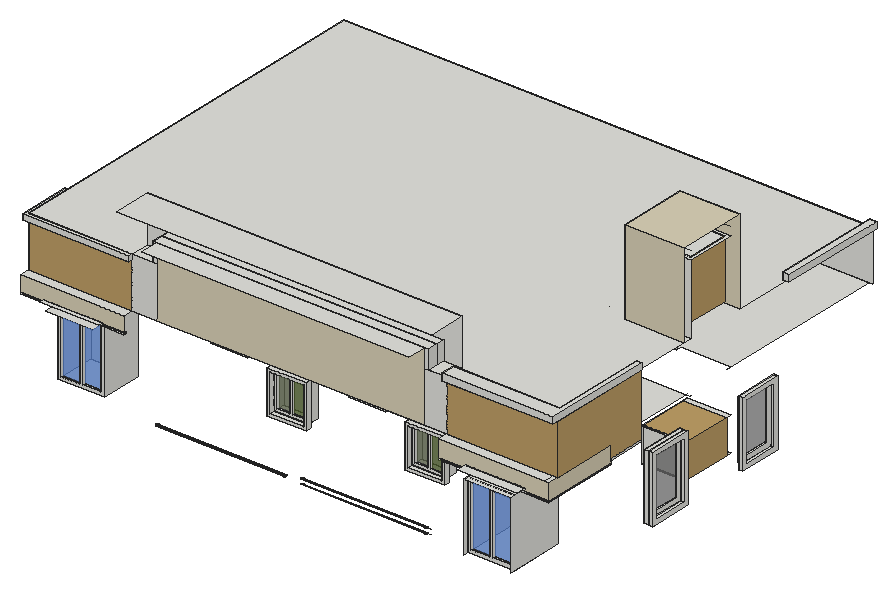
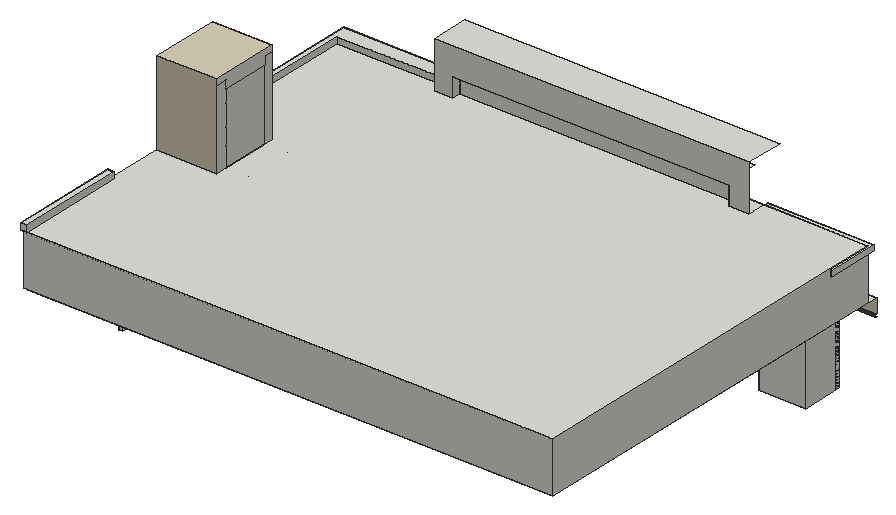
# SketchUp Ruby script. Lengths in inches.
U = 1.inch
M = Sketchup.active_model
def pt(a) = Geom::Point3d.new(a.map { |v| v * U })
def face(e, loops, mat)
  f = e.add_face(loops[0].map { |a| pt(a) })
  loops[1..].each { |l| e.add_face(l.map { |a| pt(a) }).erase! }
  f.material = f.back_material = mat if mat
  f
end
# faces: each face lists its corners as indices into pts; further lists are holes
def faces(e, pts, list, mat = nil) = list.each { |f| face(e, (f[0].is_a?(Array) ? f : [f]).map { |l| l.map { |i| pts[i] } }, mat) }
# xy, xz, yz: faces in a plane at the given z, y or x. An outline is a flat list of corners, or four numbers for a rectangle; further outlines are holes
def ring(l) = l.size == 4 ? [[l[0], l[1]], [l[2], l[1]], [l[2], l[3]], [l[0], l[3]]] : l.each_slice(2).to_a
def flat(e, list, mat, &to3) = list.each { |f| face(e, (f[0].is_a?(Array) ? f : [f]).map { |l| ring(l).map { |u, v| to3.(u, v) } }, mat) }
def xy(e, z, list, mat = nil) = flat(e, list, mat) { |x, y| [x, y, z] }
def xz(e, y, list, mat = nil) = flat(e, list, mat) { |x, z| [x, y, z] }
def yz(e, x, list, mat = nil) = flat(e, list, mat) { |y, z| [x, y, z] }
def lines(e, pts, list) = list.each { |a, b| e.add_line(pt(pts[a]), pt(pts[b])) }
# prism: a flat outline (further loops are holes) pulled along v
def prism(e, loops, v, mat = nil)
  f = face(e, loops, mat); d = Geom::Vector3d.new(v.map { |x| x * U })
  f.pushpull(f.normal.samedirection?(d) ? d.length : -d.length)
end
def box(e, o, s, mat = nil) = prism(e, [[o, [o[0] + s[0], o[1], o[2]], [o[0] + s[0], o[1] + s[1], o[2]], [o[0], o[1] + s[1], o[2]]]], [0, 0, s[2]], mat)
def at(x, y, z, deg = 0) = Geom::Transformation.translation(pt([x, y, z])) * Geom::Transformation.rotation(ORIGIN, Z_AXIS, deg.degrees)
def axes(o, x, y, z) = Geom::Transformation.new([*x, 0, *y, 0, *z, 0, *pt(o).to_a, 1])
def part(name) = M.definitions.add(name)
# library, detail: a bought-in or finely detailed component or shape, given as its bounding box
def library(name, o, s) = part(name).tap { |d| box(d.entities, o, s) }
def detail(e, o, s) = box(e.add_group.entities, o, s)
def put(e, d, t, mat = nil) = e.add_instance(d, t).tap { |i| i.material = mat if mat }
def group(e, t, mat = nil) = e.add_group.tap { |g| g.transformation = t; g.material = mat if mat }.entities
root = M.entities
M.materials.add("Generic").color = [191, 159, 103]
M.materials.add("Generic\#3").color = [218, 209, 183]
M.materials.add("[Color M06]").color = [86, 86, 86]
M.materials.add("[Translucent Glass Blue]").color = [100, 149, 237]
M.materials["[Translucent Glass Blue]"].alpha = 0.5
M.materials.add("[Translucent Glass Dark Green]").color = [62, 91, 5]
M.materials["[Translucent Glass Dark Green]"].alpha = 0.5
M.materials.add("[Translucent Glass Gray]").color = [128, 128, 128]
M.materials["[Translucent Glass Gray]"].alpha = 0.5
c1 = part("Group\#7")
xy(c1.entities,0,[[0,0,6,54.3125]])
xy(c1.entities,5.9,[[3,5.9,6,48.41]])
xy(c1.entities,81.98,[[3,5.9,6,48.41]])
xy(c1.entities,87.88,[[0,0,6,54.3125]])
xz(c1.entities,0,[[0,0,6,87.88]])
xz(c1.entities,5.9,[[3,5.9,6,81.98]])
xz(c1.entities,48.41,[[3,5.9,6,81.98]])
xz(c1.entities,54.3125,[[0,0,6,87.88]])
yz(c1.entities,0,[[0,0,54.3125,87.88]],"[Translucent Glass Gray]")
yz(c1.entities,3,[[5.9,5.9,48.41,81.98]],"[Translucent Glass Gray]")
yz(c1.entities,6,[[[0,0,54.3125,87.88],[5.9,5.9,48.41,81.98]]])
c2 = part("Group\#1")
xy(c2.entities,0,[[0,0,71.4375,6]])
xy(c2.entities,5.26,[[5.26,0,33.09,3],[38.35,0,66.18,3]])
xy(c2.entities,97.49,[[5.26,0,33.09,3],[38.35,0,66.18,3]])
xy(c2.entities,102.75,[[0,0,71.4375,6]])
xz(c2.entities,0,[[[0,0,71.4375,102.75],[38.35,5.26,66.18,97.49],[5.26,5.26,33.09,97.49]]])
xz(c2.entities,3,[[5.26,5.26,33.09,97.49],[38.35,5.26,66.18,97.49]],"[Translucent Glass Blue]")
xz(c2.entities,6,[[0,0,71.4375,102.75]],"[Translucent Glass Blue]")
yz(c2.entities,0,[[0,0,6,102.75]])
yz(c2.entities,5.26,[[0,5.26,3,97.49]])
yz(c2.entities,33.09,[[0,5.26,3,97.49]])
yz(c2.entities,38.35,[[0,5.26,3,97.49]])
yz(c2.entities,66.18,[[0,5.26,3,97.49]])
yz(c2.entities,71.4375,[[0,0,6,102.75]])
c3 = part("Group\#3")
xy(c3.entities,0,[[0,0,51.8125,6]])
xy(c3.entities,4.04,[[4.04,0,23.89,3],[27.93,0,47.77,3]])
xy(c3.entities,53.71,[[4.04,0,23.89,3],[27.93,0,47.77,3]])
xy(c3.entities,57.75,[[0,0,51.8125,6]])
xz(c3.entities,0,[[[0,0,51.8125,57.75],[4.04,4.04,23.89,53.71],[27.93,4.04,47.77,53.71]]])
xz(c3.entities,3,[[4.04,4.04,23.89,53.71],[27.93,4.04,47.77,53.71]],"[Translucent Glass Dark Green]")
xz(c3.entities,6,[[0,0,51.8125,57.75]],"[Translucent Glass Gray]")
yz(c3.entities,0,[[0,0,6,57.75]])
yz(c3.entities,4.04,[[0,4.04,3,53.71]])
yz(c3.entities,23.89,[[0,4.04,3,53.71]])
yz(c3.entities,27.93,[[0,4.04,3,53.71]])
yz(c3.entities,47.77,[[0,4.04,3,53.71]])
yz(c3.entities,51.8125,[[0,0,6,57.75]])
xy(root,918.09,[[802.875,257.24,809.375,324.36],[809.375,257.24,815.3125,324.36],[809.375,428.47,815.3125,495.59]])
xy(root,924.5,[[802.875,263.64,809.375,317.96],[809.375,263.64,815.3125,317.96],[802.875,434.88,809.375,489.19],[809.375,434.88,815.3125,489.19]])
xy(root,926.06,[[691.41,60.5625,762.85,142.1875]])
xy(root,926.27,[[49.01,83.8125,120.45,146.5625]])
xy(root,940.24,[[314.35,150.125,374.25,158.75],[524.6,150.125,584.5,158.75]])
xy(root,941.3,[[736.34,335.75,802.875,338.625],[736.34,413.6875,802.875,422.3125]])
xy(root,941.3,[[736.34,338.625,802.875,413.6875]],"Generic")
xy(root,944.28,[[318.39,150.125,370.21,158.75],[528.64,150.125,580.46,158.75],[318.39,158.75,370.21,177.1875],[528.64,158.75,580.46,177.1875]])
xy(root,993.42,[[736.34,335.75,802.875,338.625],[736.34,413.6875,802.875,422.3125]])
xy(root,993.42,[[736.34,338.625,802.875,413.6875]],"Generic")
xy(root,1002.03,[[318.39,150.125,370.21,158.75],[528.64,150.125,580.46,158.75],[318.39,158.75,370.21,177.1875],[528.64,158.75,580.46,177.1875]])
xy(root,1003,[[222.01,158.75,277.69,214.75],[432.26,158.75,487.94,214.75]])
xy(root,1006.07,[[314.35,150.125,374.25,158.75],[524.6,150.125,584.5,158.75]])
xy(root,1012.38,[[802.875,263.64,809.375,317.96],[809.375,263.64,815.3125,317.96],[802.875,434.88,809.375,489.19],[809.375,434.88,815.3125,489.19]])
xy(root,1018.78,[[802.875,257.24,809.375,324.36],[809.375,257.24,815.3125,324.36],[809.375,428.47,815.3125,495.59]])
xy(root,1028.81,[[691.41,53.22,762.85,142.1875]])
xy(root,1029.07,[[49.01,60.5625,120.45,83.8125],[49.01,83.8125,120.45,146.5625]])
xy(root,1031.12,[[641.55,68.5,682.51,69.9375],[682.51,68.5,771.75,83.8125],[771.75,68.5,809.375,69.9375],[807.9375,69.9375,809.375,185.01]])
xy(root,1033.33,[[4.1875,68.5,40.11,71.125],[129.35,68.5,162.33,71.375]])
xy(root,1034.12,[[641.55,68.5,682.51,69.9375],[771.75,68.5,809.375,69.9375],[807.9375,69.9375,809.375,185.01]])
xy(root,1036.33,[[4.1875,68.5,40.11,71.125],[129.35,68.5,162.33,71.375]])
xy(root,1037.71,[[682.51,53.22,771.75,68.5]])
xy(root,1037.97,[[40.11,60.5625,129.35,68.5],[40.11,68.5,129.35,83.8125]])
xy(root,1059,[[4.1875,68.5,162.33,83.8125],[641.55,68.5,802.875,83.8125],[802.875,68.5,809.375,83.8125],[4.1875,83.8125,4.1875,239.73,802.875,239.73,802.875,185.01,809.375,185.01,809.375,83.8125,613.23,83.8125,613.23,158.75,415.53,158.75,415.53,83.8125,391.53,83.8125,391.53,158.75,193.83,158.75,193.83,83.8125],[193.83,83.8125,391.53,158.75],
  [415.53,83.8125,613.23,158.75],[4.1875,239.73,4.1875,683.8125,802.875,683.8125,802.875,422.3125,726.91,422.3125,726.91,413.6875,709.66,413.6875,709.66,338.625,726.91,338.625,726.91,335.75,802.875,335.75,802.875,239.73],[709.66,338.625,718.29,413.6875]])
xy(root,1128.4375,[[0,77.8125,0,157.5625,4.1875,157.5625,4.1875,83.8125,162.33,83.8125,162.33,77.8125]])
xy(root,1136.625,[[641.55,73.875,811.125,83.8125],[0,77.8125,162.33,77.8125,162.33,83.8125,4.1875,83.8125,4.1875,157.5625,0,157.5625],[4.1875,83.8125,162.33,83.8125,162.33,112.625,193.83,112.625,193.83,100.0625,613.23,100.0625,613.23,112.625,641.55,112.625,641.55,95.8125,802.875,95.8125,802.875,242.76,809.375,242.76,809.375,325.3125,718.29,325.3125,718.29,431.25,809.375,431.25,809.375,518.09,804.5,518.09,804.5,683.8125,4.1875,683.8125],[162.33,83.8125,193.83,112.625],[613.23,83.8125,641.55,112.625],
  [641.55,83.8125,809.375,95.8125],[809.375,83.8125,811.125,242.76],[802.875,95.8125,809.375,242.76],[718.29,325.3125,809.375,338.625],[718.29,338.625,726.91,413.6875],
  [804.5,518.09,809.375,683.8125],[809.375,518.09,814.875,683.8125]])
xy(root,1146.5625,[[641.55,73.875,811.125,73.875,811.125,242.76,802.875,242.76,802.875,95.8125,641.55,95.8125],[804.5,518.09,814.875,683.8125]])
xy(root,1154.5625,[[723.48,343.82,804.18,408.49]],"Generic")
xy(root,1165.125,[[200.02,54.3125,607.05,83.8125],[193.83,83.8125,613.23,100.0625],[193.83,100.0625,613.23,112.625]])
xy(root,1207.3125,[[162.33,54.3125,641.55,112.625]])
xy(root,1243.75,[[[718.29,338.625,809.375,413.6875],[723.48,343.82,804.18,408.49]],[723.48,343.82,804.18,408.49]])
xy(root,1265.4375,[[718.29,325.3125,809.375,431.25]],"Generic\#3")
xz(root,68.5,[[682.51,1031.12,771.75,1034.12],[40.11,1033.33,129.35,1036.33],[682.51,1034.12,771.75,1037.71],[40.11,1036.33,129.35,1037.97]])
xz(root,68.5,[[641.55,1034.12,682.51,1034.12,682.51,1037.71,771.75,1037.71,771.75,1034.12,809.375,1034.12,809.375,1059,641.55,1059],[4.1875,1036.33,40.11,1036.33,40.11,1037.97,129.35,1037.97,129.35,1036.33,162.33,1036.33,162.33,1059,4.1875,1059]],"Generic\#3")
xz(root,69.9375,[[641.55,1031.12,682.51,1034.12],[771.75,1031.12,807.9375,1034.12]],"[Color M06]")
xz(root,71.125,[[4.1875,1033.33,40.11,1036.33]],"[Color M06]")
xz(root,71.375,[[129.35,1033.33,162.33,1036.33]],"[Color M06]")
xz(root,73.875,[[641.55,1136.625,811.125,1146.5625]])
xz(root,77.8125,[[0,1128.4375,162.33,1136.625]])
xz(root,83.8125,[[162.33,1059,200.02,1136.625],[607.05,1059,641.55,1136.625],[4.1875,1128.4375,162.33,1136.625],[193.83,1136.625,200.02,1165.125],[607.05,1136.625,613.23,1165.125]])
xz(root,83.8125,[[4.1875,1059,162.33,1128.4375],[641.55,1059,809.375,1136.625]],"Generic")
xz(root,83.8125,[[200.02,1059,607.05,1165.125]],"Generic\#3")
xz(root,95.8125,[[641.55,1136.625,802.875,1146.5625]])
xz(root,100.0625,[[193.83,1136.625,613.23,1165.125]])
xz(root,112.625,[[162.33,1136.625,162.33,1207.3125,641.55,1207.3125,641.55,1136.625,613.23,1136.625,613.23,1165.125,193.83,1165.125,193.83,1136.625]])
xz(root,142.1875,[[691.41,926.06,762.85,1028.81]])
xz(root,146.5625,[[49.01,926.27,120.45,1029.07]])
xz(root,150.125,[[[314.35,940.24,374.25,1006.07],[318.39,944.28,370.21,1002.03]],[[524.6,940.24,584.5,1006.07],[528.64,944.28,580.46,1002.03]]])
xz(root,157.5625,[[0,1128.4375,4.1875,1136.625]])
xz(root,158.75,[[[314.35,940.24,374.25,1006.07],[318.39,944.28,370.21,1002.03]],[[524.6,940.24,584.5,1006.07],[528.64,944.28,580.46,1002.03]]])
xz(root,177.1875,[[318.39,944.28,370.21,1002.03],[528.64,944.28,580.46,1002.03]])
xz(root,185.01,[[807.9375,1031.12,809.375,1034.12]])
xz(root,242.76,[[802.875,1136.625,811.125,1146.5625]])
xz(root,257.24,[[802.875,918.09,809.375,1018.78],[809.375,918.09,815.3125,1018.78]])
xz(root,263.64,[[802.875,924.5,809.375,1012.38],[809.375,924.5,815.3125,1012.38]])
xz(root,317.96,[[802.875,924.5,809.375,1012.38],[809.375,924.5,815.3125,1012.38]])
xz(root,324.36,[[802.875,918.09,809.375,1018.78],[809.375,918.09,815.3125,1018.78]])
xz(root,325.3125,[[718.29,1136.625,809.375,1265.4375]],"Generic\#3")
xz(root,338.625,[[736.34,941.3,802.875,993.42],[718.29,1059,726.91,1136.625],[718.29,1136.625,809.375,1243.75]])
xz(root,343.82,[[723.48,1154.5625,804.18,1243.75]],"Generic")
xz(root,408.49,[[723.48,1154.5625,804.18,1243.75]],"Generic")
xz(root,413.6875,[[718.29,1059,726.91,1136.625]])
xz(root,428.47,[[809.375,918.09,815.3125,1018.78]])
xz(root,431.25,[[718.29,1136.625,809.375,1265.4375]],"Generic\#3")
xz(root,434.88,[[802.875,924.5,809.375,1012.38],[809.375,924.5,815.3125,1012.38]])
xz(root,489.19,[[802.875,924.5,809.375,1012.38],[809.375,924.5,815.3125,1012.38]])
xz(root,495.59,[[809.375,918.09,815.3125,1018.78]])
xz(root,518.09,[[804.5,1136.625,814.875,1146.5625]])
xz(root,683.8125,[[4.1875,1059,809.375,1136.625],[804.5,1136.625,814.875,1146.5625]])
yz(root,0,[[77.8125,1128.4375,157.5625,1136.625]])
yz(root,4.1875,[[83.8125,1059,83.8125,1128.4375,157.5625,1128.4375,157.5625,1136.625,683.8125,1136.625,683.8125,1059],[83.8125,1128.4375,157.5625,1136.625]])
yz(root,40.11,[[68.5,1033.33,71.125,1036.33]])
yz(root,49.01,[[83.8125,926.27,146.5625,1029.07]])
yz(root,120.45,[[83.8125,926.27,146.5625,1029.07]])
yz(root,129.35,[[68.5,1033.33,71.375,1036.33]])
yz(root,162.33,[[77.8125,1128.4375,83.8125,1136.625]])
yz(root,193.83,[[83.8125,1136.625,100.0625,1165.125],[100.0625,1136.625,112.625,1165.125]])
yz(root,314.35,[[150.125,940.24,158.75,1006.07]])
yz(root,318.39,[[150.125,944.28,158.75,1002.03],[158.75,944.28,177.1875,1002.03]])
yz(root,370.21,[[150.125,944.28,158.75,1002.03],[158.75,944.28,177.1875,1002.03]])
yz(root,374.25,[[150.125,940.24,158.75,1006.07]])
yz(root,524.6,[[150.125,940.24,158.75,1006.07]])
yz(root,528.64,[[150.125,944.28,158.75,1002.03],[158.75,944.28,177.1875,1002.03]])
yz(root,580.46,[[150.125,944.28,158.75,1002.03],[158.75,944.28,177.1875,1002.03]])
yz(root,584.5,[[150.125,940.24,158.75,1006.07]])
yz(root,607.05,[[89.21,908.96,89.36,908.98,89.49,909.04,89.61,909.125,89.7,909.24,89.75,909.38,89.77,909.52,89.75,909.67,89.7,909.81,89.61,909.92,89.49,910.01,89.36,910.07,89.21,910.09,89.0625,910.07,88.93,910.01,88.8125,909.92,88.72,909.81,88.67,909.67,88.65,909.52,88.67,909.38,88.72,909.24,88.8125,909.125,88.93,909.04,89.0625,908.98],[89.21,916.4,89.36,916.42,89.49,916.47,89.61,916.5625,89.7,916.68,89.75,916.82,89.77,916.96,89.75,917.11,89.7,917.24,89.61,917.36,89.49,917.45,89.36,917.51,89.21,917.52,89.0625,917.51,88.93,917.45,88.8125,917.36,88.72,917.24,88.67,917.11,88.65,916.96,88.67,916.82,88.72,916.68,88.8125,916.5625,88.93,916.47,89.0625,916.42]])
yz(root,613.23,[[83.8125,1136.625,100.0625,1165.125],[100.0625,1136.625,112.625,1165.125]])
yz(root,641.55,[[73.875,1136.625,95.8125,1146.5625]])
yz(root,682.51,[[68.5,1031.12,69.9375,1034.12]])
yz(root,691.41,[[53.22,926.06,142.1875,1028.81]])
yz(root,718.29,[[338.625,1059,413.6875,1136.625],[325.3125,1136.625,338.625,1256.5625],[338.625,1136.625,413.6875,1243.75],[413.6875,1136.625,431.25,1256.5625],[338.625,1243.75,338.625,1256.5625,325.3125,1256.5625,325.3125,1265.4375,431.25,1265.4375,431.25,1256.5625,413.6875,1256.5625,413.6875,1243.75]])
yz(root,723.48,[[343.82,1154.5625,408.49,1243.75]])
yz(root,736.34,[[335.75,941.3,338.625,993.42],[338.625,941.3,413.6875,993.42],[413.6875,941.3,422.3125,993.42]])
yz(root,762.85,[[53.22,926.06,142.1875,1028.81]])
yz(root,771.75,[[68.5,1031.12,69.9375,1034.12]])
yz(root,802.875,[[[257.24,918.09,324.36,1018.78],[263.64,924.5,317.96,1012.38]],[335.75,941.3,338.625,993.42],[95.8125,1136.625,242.76,1146.5625]])
yz(root,802.875,[[338.625,941.3,413.6875,993.42]],"Generic")
yz(root,804.18,[[343.82,1154.5625,408.49,1243.75]],"Generic")
yz(root,804.5,[[518.09,1136.625,683.8125,1146.5625]])
yz(root,807.9375,[[69.9375,1031.12,185.01,1034.12]],"[Color M06]")
yz(root,809.375,[[[257.24,918.09,324.36,1018.78],[263.64,924.5,317.96,1012.38]],[[428.47,918.09,495.59,1018.78],[434.88,924.5,489.19,1012.38]],[185.01,1037.39,242.76,1039.96]])
yz(root,809.375,[[185.01,1039.96,242.76,1039.96,242.76,1136.625,83.8125,1136.625,83.8125,1059,185.01,1059]],"Generic")
yz(root,809.375,[[68.5,1034.12,185.01,1059]],"Generic\#3")
yz(root,811.125,[[73.875,1136.625,242.76,1146.5625]])
yz(root,814.875,[[518.09,1136.625,683.8125,1146.5625]])
yz(root,815.3125,[[[257.24,918.09,324.36,1018.78],[263.64,924.5,317.96,1012.38]],[[428.47,918.09,495.59,1018.78],[434.88,924.5,489.19,1012.38]]])
p = [[415.53,88.8125,909.125],[415.53,88.93,909.04],[607.05,88.93,909.04],[607.05,88.8125,909.125],[415.53,89.0625,908.98],[607.05,89.0625,908.98],
  [415.53,89.21,908.96],[607.05,89.21,908.96],[415.53,89.36,908.98],[607.05,89.36,908.98],[415.53,89.49,909.04],[607.05,89.49,909.04],
  [415.53,89.61,909.125],[607.05,89.61,909.125],[415.53,88.72,909.24],[607.05,88.72,909.24],[415.53,89.7,909.24],[607.05,89.7,909.24],
  [415.53,88.67,909.38],[607.05,88.67,909.38],[415.53,89.75,909.38],[607.05,89.75,909.38],[415.53,88.65,909.52],[607.05,88.65,909.52],
  [415.53,89.77,909.52],[607.05,89.77,909.52],[415.53,88.67,909.67],[607.05,88.67,909.67],[415.53,89.75,909.67],[607.05,89.75,909.67],
  [415.53,88.72,909.81],[607.05,88.72,909.81],[415.53,89.7,909.81],[607.05,89.7,909.81],[415.53,88.8125,909.92],[607.05,88.8125,909.92],
  [415.53,89.61,909.92],[607.05,89.61,909.92],[415.53,88.93,910.01],[607.05,88.93,910.01],[415.53,89.49,910.01],[607.05,89.49,910.01],
  [415.53,89.0625,910.07],[607.05,89.0625,910.07],[415.53,89.36,910.07],[607.05,89.36,910.07],[415.53,89.21,910.09],[607.05,89.21,910.09],
  [193.83,89.44,911.12],[193.83,89.73,911],[391.53,89.73,911],[391.53,89.44,911.12],[193.83,90.04,910.96],[391.53,90.04,910.96],
  [193.83,90.35,911],[391.53,90.35,911],[193.83,90.63,911.12],[391.53,90.63,911.12],[193.83,89.2,911.31],[391.53,89.2,911.31],
  [193.83,90.88,911.31],[391.53,90.88,911.31],[193.83,89.01,911.55],[391.53,89.01,911.55],[193.83,91.07,911.55],[391.53,91.07,911.55],
  [193.83,88.89,911.84],[391.53,88.89,911.84],[193.83,91.18,911.84],[391.53,91.18,911.84],[193.83,88.85,912.15],[391.53,88.85,912.15],
  [193.83,91.23,912.15],[391.53,91.23,912.15],[193.83,88.89,912.45],[391.53,88.89,912.45],[193.83,91.18,912.45],[391.53,91.18,912.45],
  [193.83,89.01,912.74],[391.53,89.01,912.74],[193.83,91.07,912.74],[391.53,91.07,912.74],[193.83,89.2,912.99],[391.53,89.2,912.99],
  [193.83,90.88,912.99],[391.53,90.88,912.99],[193.83,89.44,913.17],[391.53,89.44,913.17],[193.83,90.63,913.17],[391.53,90.63,913.17],
  [193.83,89.73,913.29],[391.53,89.73,913.29],[193.83,90.35,913.29],[391.53,90.35,913.29],[193.83,90.04,913.33],[391.53,90.04,913.33],
  [415.53,88.93,916.47],[415.53,89.0625,916.42],[607.05,89.0625,916.42],[607.05,88.93,916.47],[415.53,89.21,916.4],[607.05,89.21,916.4],
  [415.53,89.36,916.42],[607.05,89.36,916.42],[415.53,89.49,916.47],[607.05,89.49,916.47],[415.53,88.8125,916.5625],[607.05,88.8125,916.5625],
  [415.53,89.61,916.5625],[607.05,89.61,916.5625],[415.53,88.72,916.68],[607.05,88.72,916.68],[415.53,89.7,916.68],[607.05,89.7,916.68],
  [415.53,88.67,916.82],[607.05,88.67,916.82],[415.53,89.75,916.82],[607.05,89.75,916.82],[415.53,88.65,916.96],[607.05,88.65,916.96],
  [415.53,89.77,916.96],[607.05,89.77,916.96],[415.53,88.67,917.11],[607.05,88.67,917.11],[415.53,89.75,917.11],[607.05,89.75,917.11],
  [415.53,88.72,917.24],[607.05,88.72,917.24],[415.53,89.7,917.24],[607.05,89.7,917.24],[415.53,88.8125,917.36],[607.05,88.8125,917.36],
  [415.53,89.61,917.36],[607.05,89.61,917.36],[415.53,88.93,917.45],[607.05,88.93,917.45],[415.53,89.0625,917.51],[607.05,89.0625,917.51],
  [415.53,89.49,917.45],[415.53,89.36,917.51],[607.05,89.36,917.51],[607.05,89.49,917.45],[415.53,89.21,917.52],[607.05,89.21,917.52],
  [415.53,89.21,916.93],[613.23,89.21,916.93],[415.53,89.21,909.49],[613.23,89.21,909.49],[193.83,90.04,912.15],[391.53,90.04,912.15],
  [809.375,413.6875,1256.5625],[718.29,413.6875,1256.5625],[809.375,338.625,1256.5625],[718.29,338.625,1256.5625],[802.875,422.3125,1059],[802.875,413.6875,1059],
  [809.375,335.75,1059],[802.875,335.75,1059],[802.875,338.625,1059],[809.375,338.625,1059],[684.5625,413.6875,1136.625],[684.5625,413.6875,1059],
  [684.5625,338.625,1136.625],[684.5625,338.625,1059]]
faces(root,p,[[0,1,2,3],[1,4,5,2],[4,6,7,5],[6,8,9,7],[8,10,11,9],[10,12,13,11],[14,0,3,15],[12,16,17,13],
  [18,14,15,19],[16,20,21,17],[22,18,19,23],[20,24,25,21],[26,22,23,27],[24,28,29,25],[30,26,27,31],[28,32,33,29],
  [34,30,31,35],[32,36,37,33],[38,34,35,39],[36,40,41,37],[42,38,39,43],[40,44,45,41],[46,42,43,47],[44,46,47,45],
  [48,49,50,51],[49,52,53,50],[52,54,55,53],[54,56,57,55],[58,48,51,59],[56,60,61,57],[62,58,59,63],[60,64,65,61],
  [66,62,63,67],[64,68,69,65],[70,66,67,71],[68,72,73,69],[74,70,71,75],[72,76,77,73],[78,74,75,79],[76,80,81,77],
  [82,78,79,83],[80,84,85,81],[86,82,83,87],[84,88,89,85],[90,86,87,91],[88,92,93,89],[94,90,91,95],[92,94,95,93],
  [96,97,98,99],[97,100,101,98],[100,102,103,101],[102,104,105,103],[106,96,99,107],[104,108,109,105],[110,106,107,111],[108,112,113,109],
  [114,110,111,115],[112,116,117,113],[118,114,115,119],[116,120,121,117],[122,118,119,123],[120,124,125,121],[126,122,123,127],[124,128,129,125],
  [130,126,127,131],[128,132,133,129],[134,130,131,135],[136,134,135,137],[138,139,140,141],[132,138,141,133],[142,136,137,143],[139,142,143,140]])
lines(root,p,[[144,145],[146,147],[148,149],[150,151],[152,153],[154,155],[156,157],[158,157],[156,159],[160,161],[162,163]])
put(root,c1,at(803.375,434.88,924.5))
put(root,c1,at(803.375,263.64,924.5))
put(root,c2,at(691.41,60.5625,926.06))
put(root,c2,at(49.01,83.8125,926.32))
put(root,c3,at(318.39,158.75,944.28))
put(root,c3,at(528.64,158.75,944.28))
